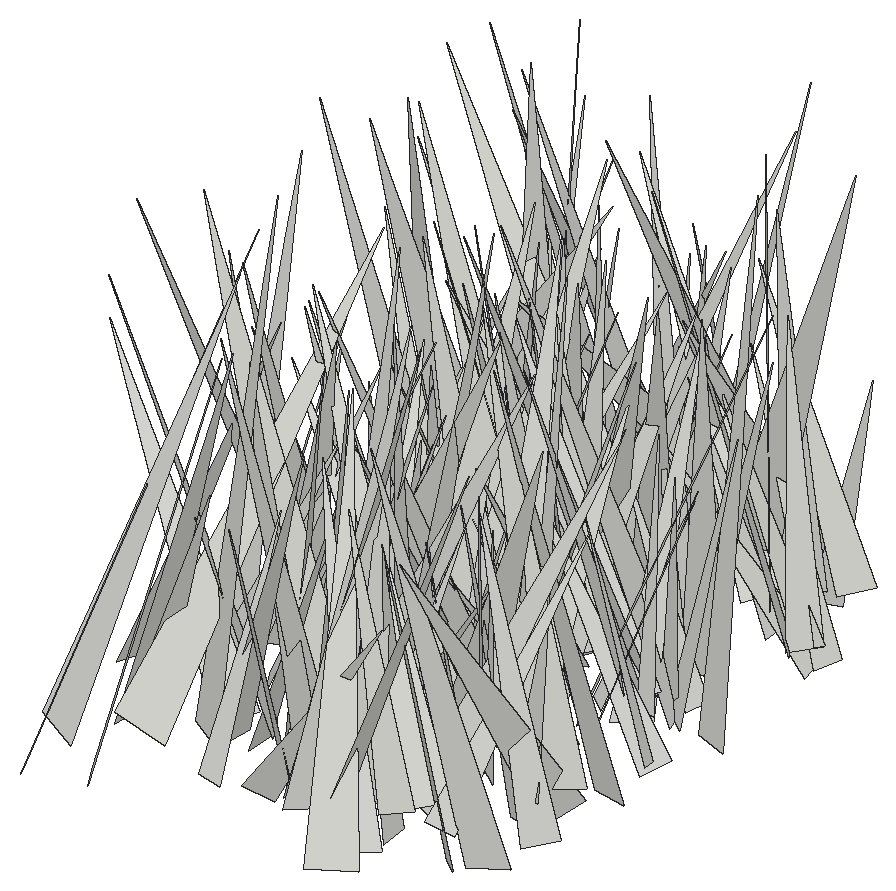
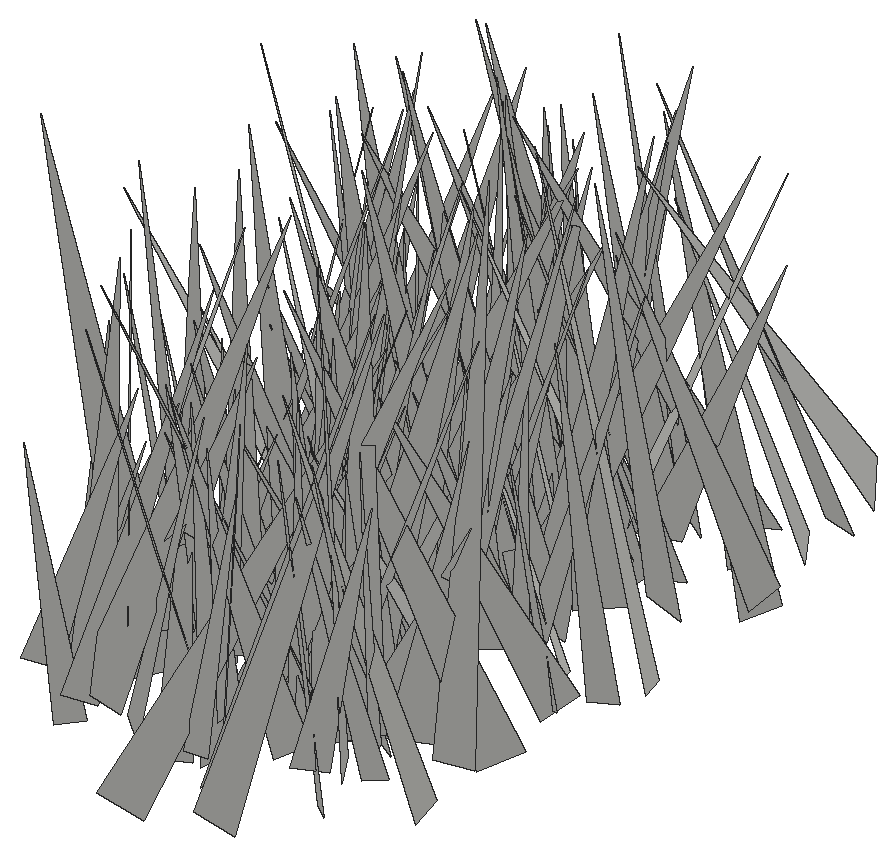
# SketchUp Ruby script. Lengths in inches.
U = 1.inch
M = Sketchup.active_model
def pt(a) = Geom::Point3d.new(a.map { |v| v * U })
def face(e, loops, mat)
  f = e.add_face(loops[0].map { |a| pt(a) })
  loops[1..].each { |l| e.add_face(l.map { |a| pt(a) }).erase! }
  f.material = f.back_material = mat if mat
  f
end
# faces: each face lists its corners as indices into pts; further lists are holes
def faces(e, pts, list, mat = nil) = list.each { |f| face(e, (f[0].is_a?(Array) ? f : [f]).map { |l| l.map { |i| pts[i] } }, mat) }
# xy, xz, yz: faces in a plane at the given z, y or x. An outline is a flat list of corners, or four numbers for a rectangle; further outlines are holes
def ring(l) = l.size == 4 ? [[l[0], l[1]], [l[2], l[1]], [l[2], l[3]], [l[0], l[3]]] : l.each_slice(2).to_a
def flat(e, list, mat, &to3) = list.each { |f| face(e, (f[0].is_a?(Array) ? f : [f]).map { |l| ring(l).map { |u, v| to3.(u, v) } }, mat) }
def xy(e, z, list, mat = nil) = flat(e, list, mat) { |x, y| [x, y, z] }
def xz(e, y, list, mat = nil) = flat(e, list, mat) { |x, z| [x, y, z] }
def yz(e, x, list, mat = nil) = flat(e, list, mat) { |y, z| [x, y, z] }
def lines(e, pts, list) = list.each { |a, b| e.add_line(pt(pts[a]), pt(pts[b])) }
# prism: a flat outline (further loops are holes) pulled along v
def prism(e, loops, v, mat = nil)
  f = face(e, loops, mat); d = Geom::Vector3d.new(v.map { |x| x * U })
  f.pushpull(f.normal.samedirection?(d) ? d.length : -d.length)
end
def box(e, o, s, mat = nil) = prism(e, [[o, [o[0] + s[0], o[1], o[2]], [o[0] + s[0], o[1] + s[1], o[2]], [o[0], o[1] + s[1], o[2]]]], [0, 0, s[2]], mat)
def at(x, y, z, deg = 0) = Geom::Transformation.translation(pt([x, y, z])) * Geom::Transformation.rotation(ORIGIN, Z_AXIS, deg.degrees)
def axes(o, x, y, z) = Geom::Transformation.new([*x, 0, *y, 0, *z, 0, *pt(o).to_a, 1])
def part(name) = M.definitions.add(name)
# library, detail: a bought-in or finely detailed component or shape, given as its bounding box
def library(name, o, s) = part(name).tap { |d| box(d.entities, o, s) }
def detail(e, o, s) = box(e.add_group.entities, o, s)
def put(e, d, t, mat = nil) = e.add_instance(d, t).tap { |i| i.material = mat if mat }
def group(e, t, mat = nil) = e.add_group.tap { |g| g.transformation = t; g.material = mat if mat }.entities
root = M.entities
c1 = part("fur_instance\#9")
p = [[0.8125,0,1.79],[0.67,-0.02,1.48],[0,-0.11,0],[0,0.11,0]]
faces(c1.entities,p,[[0,1,2,3]])
put(root,c1,axes([87.43,93.3,-27.1],[6.02676,-0.13267,0.65935],[-0.25057,-5.95995,1.09109],[-0.62414,1.1116,5.92866]))
put(root,c1,axes([91.89,92.4,-27.1],[-4.33384,4.15795,0.46311],[4.09626,4.08164,1.68703],[-0.85069,-1.52868,5.76409]))
put(root,c1,axes([89.26,95.5,-27.1],[1.99412,7.08431,1.8343],[7.27705,-2.12036,0.27805],[-0.77249,-1.68678,7.35436]))
put(root,c1,axes([88.28,106.05,-27.1],[-1.25565,-8.18969,1.33935],[-8.04493,1.53362,1.83538],[2.03567,1.00923,8.07955]))
put(root,c1,axes([89.11,86.3,-27.1],[6.66219,5.05954,0.23915],[4.47229,-6.06129,3.64695],[-2.37798,2.77537,7.52884]))
put(root,c1,axes([88.48,99.15,-28.22],[0.64184,-5.02818,1.67754],[-5.1921,-0.25617,1.21871],[1.0672,1.77778,4.9203]))
put(root,c1,axes([89.95,105.68,-27.1],[5.20163,-5.29224,1.8402],[-4.95757,-5.51713,-1.85336],[-2.61089,-0.0677,7.18539]))
put(root,c1,axes([90.23,107.08,-27.1],[-4.86729,-1.78674,2.25978],[-2.35287,5.02555,-1.09424],[1.66225,1.88173,5.06809]))
put(root,c1,axes([91.21,108.76,-27.1],[-3.33055,3.67395,0.98734],[3.8043,3.21801,0.85849],[0.0046,-1.30837,4.884]))
put(root,c1,axes([88.34,88.82,-27.1],[3.15625,6.97995,0.87784],[7.00121,-3.02246,-1.14023],[0.68808,-1.26383,7.57506]))
put(root,c1,axes([91.15,98.77,-27.1],[-2.16973,-4.86696,0.63571],[-4.9077,2.16207,-0.19771],[0.07681,0.6613,5.32503]))
put(root,c1,axes([89.54,88.79,-28.22],[5.27233,3.79468,0.9806],[3.62511,-5.34626,1.19781],[-1.48988,0.42019,6.38454]))
put(root,c1,axes([93.46,95.25,-27.1],[-3.35024,-7.10363,1.41562],[-6.97339,2.74138,-2.74705],[-1.95891,2.39017,7.35795]))
put(root,c1,axes([89.37,100.34,-28.22],[2.1321,2.91958,1.28602],[3.18698,-1.87905,-1.01782],[0.14466,-1.63367,3.46899]))
put(root,c1,axes([93.1,92.57,-27.1],[-5.86461,-3.9483,0.52207],[-3.9663,5.70596,-1.40208],[-0.36068,1.452,6.92942]))
put(root,c1,axes([92.15,101.69,-27.1],[-7.83608,-0.63477,1.59162],[-0.4911,7.96997,0.76075],[1.64165,-0.64574,7.82485]))
put(root,c1,axes([88.4375,107.06,-28.22],[6.39935,1.66924,0.57136],[1.67346,-6.42366,0.02366],[-0.55885,-0.12123,6.61343]))
put(root,c1,axes([88.23,92.48,-28.22],[7.28234,-1.08518,0.65082],[-1.04869,-7.30325,-0.44316],[-0.70811,-0.34428,7.3494]))
put(root,c1,axes([92.18,104.375,-27.1],[-2.52559,2.65872,0.46687],[2.62617,2.27215,1.26725],[-0.62447,-1.19747,3.44114]))
put(root,c1,axes([89,92.22,-27.1],[3.52002,-2.83902,0.00242],[-2.82378,-3.50072,0.47096],[0.29379,0.3681,4.49764]))
put(root,c1,axes([87.95,97.64,-28.22],[7.20484,3.15988,1.15153],[3.35999,-6.88107,-2.14053],[-0.14588,-2.42624,7.57051]))
put(root,c1,axes([89.45,108.07,-27.1],[0.33455,3.97904,1.71347],[4.11253,0.24873,-1.38056],[1.36232,-1.72801,3.74683]))
put(root,c1,axes([89.21,100.16,-28.22],[5.30796,-1.91017,1.71118],[-2.50762,-4.68997,2.54311],[-0.53734,3.01775,5.03546]))
put(root,c1,axes([92.15,104.61,-28.22],[2.16067,6.65454,0.44246],[6.23565,-2.18071,2.34697],[-2.36543,0.32979,6.59114]))
put(root,c1,axes([90.45,108.15,-27.1],[6.26613,3.81902,2.82967],[4.24719,-6.60086,-0.4964],[-2.13385,-1.92357,7.3214]))
put(root,c1,axes([93.45,105.1,-28.22],[-7.05109,-1.52018,0.70264],[-1.52291,7.08527,0.04653],[0.69669,0.10238,7.21295]))
put(root,c1,axes([93.54,99.84,-27.1],[-1.50811,5.89701,0.63499],[5.61901,1.21081,2.10069],[-1.89858,-1.1007,5.71281]))
put(root,c1,axes([90.5,100.38,-27.1],[-0.97115,-4.17934,0.95629],[-4.09852,1.19278,1.05068],[1.25838,0.65947,4.16006]))
put(root,c1,axes([87.36,105.06,-27.1],[3.63581,-6.29578,1.08718],[-5.74464,-2.67402,3.72648],[2.79605,2.69271,6.24254]))
put(root,c1,axes([92.41,96.91,-28.22],[-1.04582,-7.4675,1.55674],[-7.62212,0.96116,-0.50998],[-0.30029,1.61039,7.52311]))
put(root,c1,axes([91.29,106.58,-27.1],[6.49174,-3.69034,2.54193],[-3.75607,-6.92147,-0.45599],[-2.44375,0.83512,7.45341]))
put(root,c1,axes([90.78,108.81,-28.22],[3.62429,3.41254,1.71474],[3.78655,-3.51895,-1.00013],[-0.49783,-1.92166,4.87654]))
put(root,c1,axes([90.93,102.49,-27.1],[0.8236,-4.35079,0.44599],[-4.32851,-0.74586,0.71716],[0.62636,0.56649,4.3696]))
put(root,c1,axes([92.64,111.23,-28.22],[-1.44964,-7.72306,0.36058],[-7.72764,1.4358,-0.315],[-0.24346,0.41228,7.85162]))
put(root,c1,axes([91.01,101.9,-28.22],[4.7893,3.01055,0.30481],[2.77693,-4.59952,1.79634],[-1.20208,1.36921,5.36414]))
put(root,c1,axes([92.85,104.45,-27.1],[-4.63028,1.37895,0.71291],[1.15549,4.55932,-1.31404],[1.03661,1.07721,4.64912]))
put(root,c1,axes([94.78,107.02,-27.1],[-7.32124,-3.15954,0.71739],[-3.23761,7.2018,-1.32279],[0.12329,1.49974,7.86343]))
put(root,c1,axes([90.14,90.27,-27.1],[0.04279,8.23701,0.26485],[7.98617,0.02394,-2.03491],[2.0346,-0.26721,7.98181]))
put(root,c1,axes([89.91,94.05,-27.1],[2.31497,4.33574,1.17317],[4.28428,-1.73503,-2.04175],[1.34907,-1.93005,4.47091]))
put(root,c1,axes([91.78,91.17,-27.1],[4.31651,6.80061,2.35568],[7.01576,-4.58865,0.3914],[-1.60519,-1.76799,8.04533]))
put(root,c1,axes([93.95,102.96,-27.1],[-6.02527,4.37662,1.94606],[4.73834,5.90349,1.39383],[0.70004,-2.28907,7.31546]))
put(root,c1,axes([94.18,93.65,-27.1],[-5.61004,5.72169,2.32507],[6.16954,5.3361,1.75473],[0.28367,-2.89906,7.81865]))
put(root,c1,axes([91.6,99.12,-27.1],[-0.33332,4.6985,0.41104],[4.65173,0.39553,-0.74898],[0.77866,-0.35159,4.65038]))
put(root,c1,axes([95.36,105.56,-27.1],[-7.15301,3.97515,0.71331],[4.02795,6.91641,1.848],[-0.2937,-1.95899,7.97197]))
put(root,c1,axes([90.27,98.55,-28.22],[3.77978,1.93812,0.15141],[1.88384,-3.56988,-1.33157],[0.48001,-1.25124,4.0336]))
put(root,c1,axes([94.38,109.125,-28.22],[-7.47727,-2.4998,1.10622],[-2.44373,7.5564,0.55783],[1.22512,-0.18436,7.86431]))
put(root,c1,axes([92.45,103.65,-27.1],[4.52412,1.43506,1.852],[1.32361,-4.8885,0.5546],[-1.93323,0.01133,4.71375]))
put(root,c1,axes([90.53,94.05,-27.1],[3.62784,4.7769,0.79864],[4.78599,-3.38301,-1.50576],[0.74217,-1.53438,5.80626]))
put(root,c1,axes([94.5625,97.875,-28.22],[-6.22564,-1.43503,0.72375],[-1.44178,6.26598,0.02194],[0.71021,0.14105,6.38885]))
put(root,c1,axes([90.93,105.11,-27.1],[2.90459,3.11145,0.76807],[3.13189,-2.53582,-1.57117],[0.67994,-1.61126,3.9559]))
put(root,c1,axes([91.51,100.24,-27.1],[1.83451,-3.56347,0.05806],[-3.52397,-1.80394,0.62811],[0.53227,0.33851,3.95843]))
put(root,c1,axes([90.62,96.59,-27.1],[3.94338,-5.9757,0.15667],[-5.94055,-3.89659,0.90015],[0.66588,0.62564,7.10275]))
put(root,c1,axes([95.38,91.52,-28.22],[1.68916,7.29229,2.94864],[7.0223,-2.75681,2.79508],[-3.5439,-1.98689,6.94394]))
put(root,c1,axes([93.7,96.125,-28.22],[-1.75814,5.2069,0.13379],[5.20853,1.75836,0.01288],[0.0306,-0.13088,5.4957]))
put(root,c1,axes([95,101.29,-28.22],[-3.10953,-4.00727,0.37973],[-3.98696,3.00024,-0.98706],[-0.55366,0.90108,4.97525]))
put(root,c1,axes([91.875,94.9,-28.22],[6.17791,2.14602,1.95241],[2.61385,-6.11017,-1.55482],[-1.25898,-2.15507,6.35252]))
put(root,c1,axes([91.88,97.88,-27.1],[3.27603,2.91205,0.73309],[2.99826,-3.11162,-1.03833],[0.1671,-1.26001,4.25844]))
put(root,c1,axes([92,93.29,-28.22],[4.64255,0.07182,0.51653],[0.0806,-4.67045,-0.07504],[-0.51523,-0.08349,4.6425]))
put(root,c1,axes([91.31,94.46,-27.1],[5.4364,3.24485,0.19999],[3.25087,-5.4295,-0.27539],[-0.03035,-0.33899,6.32516]))
put(root,c1,axes([94.55,96.64,-27.1],[0.42808,-6.23217,1.75974],[-6.34467,-0.7568,-1.13683],[-1.29687,1.64535,6.14254]))
put(root,c1,axes([95.11,92.58,-28.22],[-1.73003,-6.76572,2.01517],[-7.01807,1.42401,-1.24409],[-0.76325,2.2419,6.8717]))
put(root,c1,axes([93.5,104.56,-28.22],[0.33576,5.45677,2.6197],[6.05197,-0.25349,-0.24764],[0.11336,-2.62894,5.46148]))
put(root,c1,axes([93.46,89.2,-27.1],[0.89706,4.01856,0.51185],[4.05094,-0.89322,-0.08685],[-0.02607,-0.51851,4.11655]))
put(root,c1,axes([94.67,104.9375,-28.22],[-5.66532,-0.50223,1.85308],[-0.88322,5.80808,-1.12609],[1.70472,1.34012,5.57494]))
put(root,c1,axes([94.8,105.01,-27.1],[-4.25051,-1.02119,0.70994],[-0.79222,4.17184,1.25768],[0.95876,-1.08007,4.18663]))
put(root,c1,axes([92.52,103.67,-27.1],[1.65691,4.63189,0.02775],[4.518,-1.60961,-1.09423],[1.0212,-0.39403,4.79608]))
put(root,c1,axes([93.37,101.07,-27.1],[3.56009,0.21869,0.65734],[0.01468,-3.46445,1.07311],[-0.69261,1.05069,3.40155]))
put(root,c1,axes([95.18,99.8125,-28.22],[-5.98098,3.27291,2.42019],[3.72115,6.13978,0.89298],[1.64993,-1.98304,6.75918]))
put(root,c1,axes([94.24,110.03,-27.1],[-0.05824,-3.81958,0.55077],[-3.85535,0.08183,0.15984],[0.16986,0.54776,3.81668]))
put(root,c1,axes([95.28,112.08,-28.22],[5.32765,-5.22538,0.29084],[-4.03169,-4.36253,-4.52625],[-3.33686,-3.07194,5.93309]))
put(root,c1,axes([92.24,108.26,-27.1],[4.93305,-2.19664,0.15391],[-2.18894,-4.85066,0.92924],[0.23965,0.9109,5.31946]))
put(root,c1,axes([94.625,91.41,-28.22],[-2.78076,-3.999,1.01738],[-3.97731,2.92434,0.62365],[1.09912,0.46468,4.83071]))
put(root,c1,axes([94.88,102.64,-28.22],[-2.27159,-6.08211,1.19958],[-6.16809,2.34544,0.21162],[0.62109,1.04786,6.48903]))
put(root,c1,axes([92.5,91.38,-27.1],[6.03259,-1.06555,0.38284],[-1.02373,-6.01977,-0.62323],[-0.48366,-0.54868,6.09418]))
put(root,c1,axes([95.65,103.51,-27.1],[-3.44021,1.49763,0.22694],[1.46636,3.43395,-0.43273],[0.37973,0.30751,3.72702]))
put(root,c1,axes([97.37,94.36,-27.1],[-4.10469,4.34568,0.4298],[4.19686,3.76273,2.03626],[-1.20665,-1.6956,5.62024]))
put(root,c1,axes([94.99,107.82,-27.1],[-3.86454,-2.68359,1.87384],[-2.96857,4.09497,-0.25773],[1.3786,1.29506,4.69786]))
put(root,c1,axes([92.9,105.43,-28.22],[3.73638,-5.69312,0.32255],[-5.69521,-3.70663,0.54933],[0.28337,0.57053,6.78752]))
put(root,c1,axes([93.53,104.07,-28.22],[4.12034,-0.14152,0.59374],[0.17297,-3.61498,-2.06197],[-0.58535,-2.06437,3.57009]))
put(root,c1,axes([93.79,93.66,-28.22],[6.17707,1.48648,1.9777],[1.80034,-6.34915,-0.85095],[-1.69697,-1.32504,6.29616]))
put(root,c1,axes([94.74,103.88,-28.22],[4.88657,-1.90502,2.44295],[-2.30886,-5.28158,0.49977],[-2.06549,1.39696,5.22091]))
put(root,c1,axes([94.57,93.65,-28.22],[2.51079,7.35519,2.45383],[7.71335,-2.63218,-0.00261],[-0.79014,-2.32314,7.77193]))
put(root,c1,axes([94.16,97.81,-28.22],[-1.03239,7.59334,1.92082],[7.72051,1.31303,-1.04105],[1.31985,-1.74108,7.59215]))
put(root,c1,axes([93.89,101.93,-27.1],[3.66443,-1.25509,0.51627],[-1.25966,-3.69872,-0.05095],[-0.50503,0.11865,3.87307]))
put(root,c1,axes([94.93,107.69,-27.1],[4.11345,0.18865,1.81103],[0.00918,-4.47631,0.44541],[-1.8208,0.4036,4.09361]))
put(root,c1,axes([97.22,103.26,-27.1],[-5.99784,0.36822,0.31916],[0.44096,5.77868,1.61988],[0.20737,-1.63795,5.78668]))
put(root,c1,axes([93.84,99.71,-28.22],[0.26684,4.21608,0.5662],[4.07293,-0.08948,-1.25314],[1.22767,-0.6195,4.03438]))
put(root,c1,axes([94.28,100.11,-27.1],[-1.25446,7.26591,1.58891],[7.27727,1.53186,-1.25954],[1.53602,-1.32352,7.26503]))
put(root,c1,axes([93.03,95.16,-27.1],[5.29628,3.42643,1.15131],[3.61426,-4.98862,-1.7797],[0.0553,-2.11891,6.05175]))
put(root,c1,axes([95.92,103.0625,-27.1],[-4.49863,-0.46507,1.40367],[-0.60193,4.68178,-0.37796],[1.35065,0.53749,4.50678]))
put(root,c1,axes([92.05,104.55,-27.1],[6.81977,1.54998,0.06465],[1.44583,-6.24479,-2.79788],[0.56233,-2.74155,6.40965]))
put(root,c1,axes([96,95.54,-27.1],[1.13242,-3.28388,1.61058],[-3.44754,-1.52145,-0.67814],[-1.2216,1.24962,3.40681]))
put(root,c1,axes([97.63,104.85,-28.22],[-7.72963,0.57294,0.92033],[0.30078,7.49944,-2.14251],[1.04153,2.08628,7.44883]))
put(root,c1,axes([98.25,96.42,-27.1],[-2.1287,-6.56011,1.58213],[-6.38568,1.42177,-2.69649],[-2.18201,2.23898,6.34786]))
put(root,c1,axes([94.85,108.4,-28.22],[5.23095,-0.44242,1.6949],[-0.413,-5.49862,-0.16069],[-1.70231,-0.02548,5.24716]))
put(root,c1,axes([95.12,97.58,-28.22],[3.76197,3.17485,0.58422],[2.97684,-3.75885,1.25811],[-1.24876,0.60394,4.75913]))
put(root,c1,axes([96.27,103.5,-28.22],[1.61464,-3.26071,0.69447],[-2.99454,-1.75765,-1.29032],[-1.46534,-0.00102,3.40211]))
put(root,c1,axes([97.68,100.23,-28.22],[-5.67662,-5.13617,1.32256],[-5.29359,5.60645,-0.94818],[0.32758,1.59402,7.59639]))
put(root,c1,axes([96.31,97.54,-27.1],[-1.09873,-5.30096,0.04279],[-5.29764,1.09638,-0.20521],[-0.19227,0.08352,5.40974]))
put(root,c1,axes([94.63,92.17,-27.1],[5.61379,-0.0924,1.25595],[-0.17391,-5.73971,0.3551],[-1.24727,0.38445,5.60331]))
put(root,c1,axes([93.68,104.83,-28.22],[4.66085,6.54813,0.11631],[6.5407,-4.64683,-0.4912],[0.3329,-0.37945,8.02249]))
put(root,c1,axes([92.34,97.24,-27.1],[1.4912,-7.63112,1.5604],[-7.07021,-0.65953,3.53123],[3.26816,2.05513,6.92734]))
put(root,c1,axes([95.89,94.99,-28.22],[-6.46976,-1.55499,2.98827],[-1.52534,7.12153,0.40334],[3.00351,0.26714,6.64177]))
put(root,c1,axes([99.05,91.77,-27.1],[-3.57557,6.64036,0.56629],[6.42877,3.26724,2.27945],[-1.75672,-1.55901,7.1891]))
put(root,c1,axes([95.93,91.93,-27.1],[-2.4957,-1.61977,2.11338],[-2.18018,2.90599,-0.34732],[1.52869,1.50005,2.95492]))
put(root,c1,axes([93.75,91,-28.22],[2.63596,-3.80697,0.02165],[-3.40971,-2.34911,2.07299],[1.69332,1.196,4.14053]))
put(root,c1,axes([94.35,105.27,-28.22],[0.05129,-4.93553,2.34933],[-4.99892,0.90807,2.01684],[2.21125,2.16734,4.50493]))
put(root,c1,axes([98.99,106.99,-27.1],[-4.99082,4.3261,0.4502],[4.29852,4.80129,1.51542],[-0.66378,-1.43477,6.4286]))
put(root,c1,axes([97.76,108.4375,-28.22],[-3.65286,-4.07637,1.60167],[-4.37583,3.48496,-1.11027],[0.18514,1.94004,5.3598]))
put(root,c1,axes([95.32,104.76,-28.22],[4.63443,1.21877,0.59299],[1.09033,-4.6073,0.94811],[-0.80513,0.77609,4.69728]))
put(root,c1,axes([96.39,106.72,-28.22],[4.61652,6.22378,1.13894],[6.03614,-4.75491,1.51682],[-1.89675,0.0163,7.59914]))
put(root,c1,axes([98.04,90.17,-28.22],[-2.8304,4.89567,0.80261],[4.94903,2.72215,0.8485],[-0.34477,-1.11592,5.59096]))
put(root,c1,axes([97.34,100.68,-27.1],[-0.13278,-3.81265,0.23397],[-3.74221,0.08288,-0.77308],[-0.76609,0.25594,3.73581]))
put(root,c1,axes([97.21,101.59,-27.1],[-4.02078,2.93374,1.78068],[3.22926,4.16274,0.43339],[1.1617,-1.41743,4.95839]))
put(root,c1,axes([95.95,106.73,-27.1],[4.38322,-1.64948,1.59394],[-1.93146,-4.50849,0.64578],[-1.2373,1.19448,4.63858]))
put(root,c1,axes([95.75,109.14,-28.22],[1.95757,-4.55386,0.31612],[-4.56359,-1.94437,0.25034],[0.10577,0.38911,4.95045]))
put(root,c1,axes([98.93,98.61,-28.22],[-2.6027,-3.00196,0.39616],[-2.70686,2.07255,-2.07851],[-1.35707,1.62343,3.38609]))
put(root,c1,axes([96.56,100.01,-28.22],[-2.93741,-3.09466,0.01129],[-2.71699,2.58635,2.03327],[1.48156,-1.39259,3.75115]))
put(root,c1,axes([98.32,109.3125,-27.1],[-0.28332,-7.79704,0.77926],[-7.68212,0.12267,-1.56569],[-1.54472,0.82004,7.64347]))
put(root,c1,axes([95.47,93.13,-28.22],[3.8069,0.05751,0.20355],[-0.0416,-3.39391,1.73693],[-0.20739,1.73647,3.38805]))
put(root,c1,axes([97.61,99.58,-27.1],[5.36084,-0.19835,3.29768],[0.06393,-6.27827,-0.48156],[-3.30302,-0.44345,5.34285]))
put(root,c1,axes([98.21,97.9,-28.22],[3.70498,4.05955,2.96614],[3.93602,-4.63444,1.42637],[-3.1282,-1.02317,5.30776]))
put(root,c1,axes([95.58,90.41,-27.1],[6.99973,1.86447,1.44835],[1.77883,-7.14461,0.6004],[-1.55233,0.22015,7.21886]))
put(root,c1,axes([98.03,88.89,-28.22],[-3.98192,5.65644,1.02142],[5.69703,4.04883,-0.21229],[0.76316,-0.7113,6.91418]))
put(root,c1,axes([94.79,92.1875,-28.22],[6.18283,-3.26103,2.17206],[-3.91127,-5.37775,3.05962],[-0.2327,3.74499,6.28493]))
put(root,c1,axes([97.29,92.59,-27.1],[-7.34355,0.30763,3.29021],[-0.75169,7.65215,-2.39318],[3.21793,2.48952,6.94946]))
put(root,c1,axes([96.61,89.65,-27.1],[6.53232,-2.04401,3.08815],[-2.89411,-6.72439,1.67109],[-2.31057,2.64395,6.63752]))
put(root,c1,axes([98.21,91.47,-28.22],[-5.34365,-1.01248,1.41227],[-1.15776,5.47992,-0.452],[1.29585,0.72082,5.4199]))
put(root,c1,axes([97.9,94.37,-28.22],[-4.24869,-0.73201,1.00331],[-0.4187,4.21079,1.29914],[1.16925,-1.15205,4.11089]))
put(root,c1,axes([96.6,93.74,-28.22],[4.79188,-1.27621,1.00499],[-1.01396,-4.79557,-1.25507],[-1.26909,-0.98723,4.79746]))
put(root,c1,axes([99.59,100.65,-27.1],[-2.75065,-6.97463,1.22589],[-6.99898,2.47729,-1.60986],[-1.07823,1.71227,7.32256]))
put(root,c1,axes([97.67,90.8125,-27.1],[4.97353,-2.18793,2.98402],[-2.79783,-5.49524,0.634],[-2.42149,1.85546,5.39639]))
put(root,c1,axes([99.84,100.28,-27.1],[-3.57331,4.48467,0.98446],[4.4978,3.16833,1.89248],[-0.92266,-1.92337,5.41289]))
put(root,c1,axes([98.25,99.75,-28.22],[-4.69837,-4.55111,2.1601],[-4.81656,4.92378,-0.10244],[1.47629,1.58022,6.5404]))
put(root,c1,axes([96.69,97.85,-28.22],[4.77629,1.47467,0.59608],[1.29577,-4.70156,1.24867],[-0.92247,1.03128,4.84029]))
put(root,c1,axes([98.6875,90.99,-27.1],[-2.55012,3.64542,1.48438],[3.93085,2.44958,0.73729],[0.20222,-1.64502,4.38733]))
put(root,c1,axes([97.25,91.52,-27.1],[1.39427,3.92432,0.17719],[3.92808,-1.39069,-0.10895],[0.04345,-0.20342,4.16322]))
put(root,c1,axes([99.97,102.02,-28.22],[-7.76303,-2.55675,1.09489],[-2.43873,7.81802,0.96517],[1.33728,-0.58482,8.11604]))
put(root,c1,axes([96.26,100.66,-28.22],[0.24671,6.36494,1.6516],[6.30189,0.24313,-1.87833],[1.87786,-1.65213,6.08648]))
put(root,c1,axes([98.41,94.57,-28.22],[-3.36264,-2.39418,1.21792],[-2.41208,3.55006,0.31902],[1.18208,0.43333,4.11555]))
put(root,c1,axes([99.47,96.89,-27.1],[-5.53788,-5.2946,2.37412],[-5.70348,5.57065,-0.88067],[1.06751,2.29618,7.61087]))
put(root,c1,axes([95.94,102.86,-28.22],[7.12513,-3.29011,0.44393],[-3.26274,-7.13377,-0.50321],[-0.6135,-0.27186,7.83192]))
put(root,c1,axes([98.56,95.6875,-27.1],[-2.23719,7.0676,1.63885],[7.20712,2.3619,-0.34736],[0.83319,-1.45336,7.40509]))
put(root,c1,axes([96.71,104.84,-27.1],[1.84605,-6.6162,0.27609],[-6.51912,-1.76548,1.28157],[1.16252,0.60597,6.74831]))
put(root,c1,axes([100.22,102.42,-28.22],[-3.79909,0.62191,0.11225],[0.62576,3.79759,0.13861],[0.08831,-0.15497,3.84716]))
put(root,c1,axes([97.36,89.83,-27.1],[5.64038,0.84844,0.8162],[0.68974,-5.61874,1.07421],[-0.95409,0.95384,5.60177]))
put(root,c1,axes([98.69,109.65,-27.1],[5.3138,-2.81187,1.14067],[-1.98861,-4.96443,-2.9739],[-2.29198,-2.2118,5.22484]))
put(root,c1,axes([98.47,97.15,-27.1],[-0.0626,5.05917,0.30688],[5.04763,0.09003,-0.45456],[0.45914,-0.29998,5.03909]))
put(root,c1,axes([99.23,102.8125,-28.22],[0.08392,3.77547,1.67654],[4.10941,-0.2474,0.35143],[-0.42151,-1.66031,3.76001]))
put(root,c1,axes([97.9,100.86,-28.22],[2.19151,2.85606,0.09461],[2.85445,-2.18225,-0.24214],[0.13471,-0.22234,3.59182]))
put(root,c1,axes([99.19,106.91,-27.1],[4.97701,4.02381,2.97396],[4.34378,-5.5566,0.24873],[-2.48337,-1.65505,6.3953]))
put(root,c1,axes([98.06,97.16,-28.22],[1.68114,-3.92704,0.2758],[-3.91607,-1.63754,0.5539],[0.40264,0.46985,4.23569]))
put(root,c1,axes([100.3125,94.29,-28.22],[-2.6227,-3.62693,1.52989],[-3.9333,2.34177,-1.19122],[-0.15598,1.93268,4.31442]))
put(root,c1,axes([100.51,105.51,-27.1],[-3.97846,-0.22397,0.26493],[-0.21326,3.98441,0.16592],[0.27363,-0.15114,3.9813]))
put(root,c1,axes([100.46,91.125,-28.22],[-3.38469,-3.26483,1.22467],[-3.48648,3.19729,-1.11215],[0.05857,1.65326,4.56929]))
put(root,c1,axes([101.33,105.1,-27.1],[-5.74367,-4.09689,1.01684],[-4.21686,5.6466,-1.0688],[0.19121,1.46278,6.97366]))
put(root,c1,axes([99.35,100.55,-28.22],[-4.32625,3.6169,1.13686],[3.35652,4.45591,-1.40339],[1.76301,0.39209,5.46158]))
put(root,c1,axes([98.6875,94.78,-27.1],[3.47548,2.68418,2.07766],[3.24177,-3.50628,-0.89294],[-1.00618,-2.02524,4.29959]))
put(root,c1,axes([100.84,108.7,-27.1],[-3.29735,3.76242,1.32483],[3.9802,2.99017,1.41439],[-0.2628,-1.92005,4.79874]))
put(root,c1,axes([99.375,94.1875,-27.1],[-2.0645,-2.99831,1.70133],[-3.28642,2.31061,0.08412],[1.04107,1.34824,3.63936]))
put(root,c1,axes([99.51,108.01,-27.1],[1.40139,-5.88916,2.09043],[-6.21682,-1.53152,-0.14692],[-0.635,1.99706,6.05182]))
put(root,c1,axes([101.37,94.91,-27.1],[-2.35431,6.5098,1.98677],[6.74258,1.94391,1.62058],[-0.92858,-2.38982,6.73008]))
put(root,c1,axes([101.46,99,-28.22],[-4.14397,2.00475,0.46664],[2.04964,3.92263,1.34951],[-0.1891,-1.41534,4.40117]))
put(root,c1,axes([96.75,96.19,-28.22],[3.43044,-6.71204,0.2285],[-6.5076,-3.25868,1.97581],[1.6598,1.09595,7.27431]))
put(root,c1,axes([101.32,106.27,-28.22],[-4.59032,-0.23962,0.17171],[-0.16134,4.28449,1.66587],[0.24672,-1.65642,4.28408]))
put(root,c1,axes([101.56,106.53,-28.22],[-4.67921,0.76999,0.1435],[0.76372,4.67821,-0.1991],[0.17382,0.17327,4.73796]))
put(root,c1,axes([101.38,91.68,-28.22],[0.21483,-6.37799,2.26736],[-6.52313,-0.80094,-1.63496],[-1.80789,2.13204,6.16862]))
put(root,c1,axes([100.98,93.89,-27.1],[3.07038,6.62387,1.59445],[6.28566,-3.42873,2.13997],[-2.62838,-0.46188,6.98022]))
put(root,c1,axes([100.25,99.72,-27.1],[-5.41835,-3.58553,1.38238],[-3.2455,5.54933,1.6725],[2.0576,-0.68883,6.27832]))
put(root,c1,axes([100.51,99.74,-27.1],[1.055,3.81063,1.04337],[3.83467,-1.24762,0.6792],[-0.95124,-0.80317,3.89521]))
put(root,c1,axes([99.22,103.92,-28.22],[0.93072,-6.54849,1.55591],[-6.7031,-0.75944,0.81335],[0.60996,1.64631,6.5641]))
put(root,c1,axes([99.71,101.81,-28.22],[-1.12295,-3.74744,1.45837],[-3.89173,1.39395,0.58526],[1.01223,1.20198,3.86805]))
put(root,c1,axes([101.49,96.9,-28.22],[-2.51805,-6.35566,1.6356],[-6.55451,2.34778,-0.96776],[-0.32873,1.87181,6.76746]))
put(root,c1,axes([101.83,105.47,-27.1],[-1.39517,3.65073,1.37856],[3.73252,0.82124,1.60268],[-1.13865,-1.78115,3.56451]))
put(root,c1,axes([97.57,97.31,-27.1],[6.19787,3.91116,1.13836],[4.069,-5.84754,-2.06304],[0.19042,-2.34857,7.0324]))
put(root,c1,axes([97.88,93.15,-28.22],[1.82211,6.46965,0.85286],[6.26515,-1.48669,-2.10749],[1.8253,-1.35544,6.38239]))
put(root,c1,axes([99.33,109.24,-28.22],[2.40925,-3.29701,1.00546],[-3.44676,-2.29271,0.74099],[0.03277,1.24857,4.01568]))
put(root,c1,axes([98.9,104.61,-27.1],[3.06956,3.90435,1.71137],[4.25532,-2.68017,-1.51785],[0.25498,-2.27325,4.72887]))
put(root,c1,axes([97.97,107.12,-27.1],[6.25642,-5.32962,1.03257],[-5.42827,-6.12142,1.29455],[0.06986,1.65444,8.11614]))
put(root,c1,axes([100.18,91.04,-27.1],[-3.33289,3.23483,0.32122],[2.5841,2.91556,-2.549],[1.97223,1.64647,3.88264]))
put(root,c1,axes([101.66,93.65,-28.22],[-3.61147,3.35043,1.62323],[3.67501,3.56996,0.80783],[0.59541,-1.71259,4.85958]))
put(root,c1,axes([101.08,95.4,-28.22],[4.98513,-4.06782,0.78587],[-3.3159,-4.65458,-3.05875],[-2.48386,-1.95039,5.66063]))
put(root,c1,axes([99.24,98.42,-27.1],[5.73522,3.47371,0.17785],[3.39582,-5.66618,1.16354],[-0.75282,0.90483,6.60345]))
put(root,c1,axes([102.42,97.51,-27.1],[-3.43885,-1.25141,0.28396],[-1.28081,3.29756,-0.97876],[-0.07859,1.01608,3.52615]))
put(root,c1,axes([100.14,101.48,-28.22],[2.5994,3.80823,1.24151],[3.99906,-2.55122,-0.54734],[-0.2268,-1.33772,4.57819]))
put(root,c1,axes([101.74,105.27,-27.1],[-4.02288,2.74208,1.38872],[2.85785,4.17888,0.02734],[1.13147,-0.80565,4.86845]))
put(root,c1,axes([100.33,97.5,-27.1],[3.37937,2.22818,0.23171],[2.15143,-3.34494,0.78826],[-0.62436,0.53406,3.97033]))
put(root,c1,axes([101.8,101.04,-28.22],[3.45024,7.01244,2.07893],[6.95776,-3.8555,1.45774],[-2.25516,-1.1667,7.67811]))
